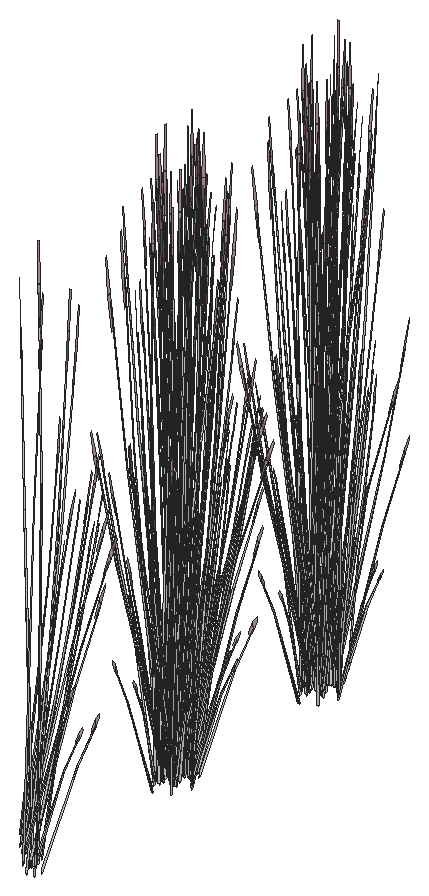
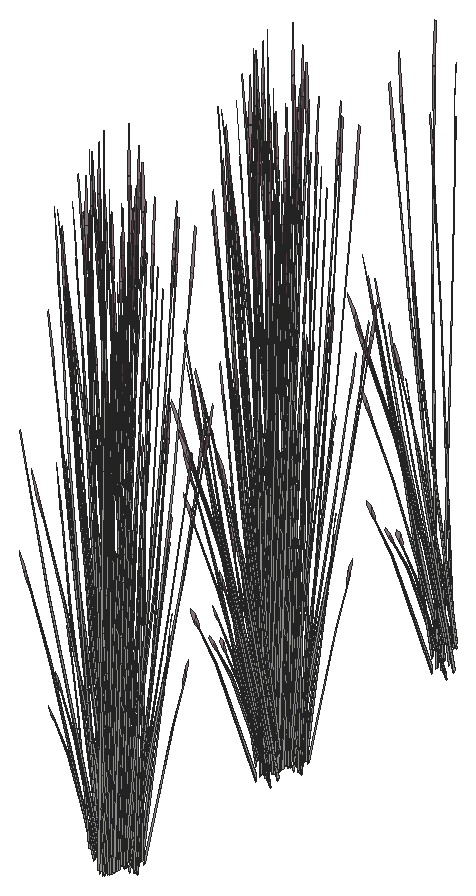
# SketchUp Ruby script. Lengths in inches.
U = 1.inch
M = Sketchup.active_model
def pt(a) = Geom::Point3d.new(a.map { |v| v * U })
def face(e, loops, mat)
  f = e.add_face(loops[0].map { |a| pt(a) })
  loops[1..].each { |l| e.add_face(l.map { |a| pt(a) }).erase! }
  f.material = f.back_material = mat if mat
  f
end
# faces: each face lists its corners as indices into pts; further lists are holes
def faces(e, pts, list, mat = nil) = list.each { |f| face(e, (f[0].is_a?(Array) ? f : [f]).map { |l| l.map { |i| pts[i] } }, mat) }
# xy, xz, yz: faces in a plane at the given z, y or x. An outline is a flat list of corners, or four numbers for a rectangle; further outlines are holes
def ring(l) = l.size == 4 ? [[l[0], l[1]], [l[2], l[1]], [l[2], l[3]], [l[0], l[3]]] : l.each_slice(2).to_a
def flat(e, list, mat, &to3) = list.each { |f| face(e, (f[0].is_a?(Array) ? f : [f]).map { |l| ring(l).map { |u, v| to3.(u, v) } }, mat) }
def xy(e, z, list, mat = nil) = flat(e, list, mat) { |x, y| [x, y, z] }
def xz(e, y, list, mat = nil) = flat(e, list, mat) { |x, z| [x, y, z] }
def yz(e, x, list, mat = nil) = flat(e, list, mat) { |y, z| [x, y, z] }
def lines(e, pts, list) = list.each { |a, b| e.add_line(pt(pts[a]), pt(pts[b])) }
# prism: a flat outline (further loops are holes) pulled along v
def prism(e, loops, v, mat = nil)
  f = face(e, loops, mat); d = Geom::Vector3d.new(v.map { |x| x * U })
  f.pushpull(f.normal.samedirection?(d) ? d.length : -d.length)
end
def box(e, o, s, mat = nil) = prism(e, [[o, [o[0] + s[0], o[1], o[2]], [o[0] + s[0], o[1] + s[1], o[2]], [o[0], o[1] + s[1], o[2]]]], [0, 0, s[2]], mat)
def at(x, y, z, deg = 0) = Geom::Transformation.translation(pt([x, y, z])) * Geom::Transformation.rotation(ORIGIN, Z_AXIS, deg.degrees)
def axes(o, x, y, z) = Geom::Transformation.new([*x, 0, *y, 0, *z, 0, *pt(o).to_a, 1])
def part(name) = M.definitions.add(name)
# library, detail: a bought-in or finely detailed component or shape, given as its bounding box
def library(name, o, s) = part(name).tap { |d| box(d.entities, o, s) }
def detail(e, o, s) = box(e.add_group.entities, o, s)
def put(e, d, t, mat = nil) = e.add_instance(d, t).tap { |i| i.material = mat if mat }
def group(e, t, mat = nil) = e.add_group.tap { |g| g.transformation = t; g.material = mat if mat }.entities
root = M.entities
M.materials.add("LightPink_Translucent").color = [144, 107, 117]
M.materials["LightPink_Translucent"].alpha = 0.75
c1 = part("blade")
p = [[2.15,0.21,22],[0,0.17,0],[0.09,0.45,0],[2.18,0.31,22],[2.29,0.31,22],[0.38,0.45,0],
  [2.48,0.24,33],[2.49,0.24,33],[2.48,0.22,33]]
faces(c1.entities,p,[[0,1,2,3],[4,5,2,3],[6,3,4,7],[8,0,3,6]])
c2 = part("seeds")
p = [[0.3,-0.1,1.38],[-0.01,-0.03,1.59],[-0.01,-0.03,0.03],[0.14,-0.07,-0.07],[0.29,-0.03,3],[0.15,0.01,3.11]]
faces(c2.entities,p,[[0,1,2,3],[1,0,4,5]],"LightPink_Translucent")
c3 = part("blade with seeds")
put(c3.entities,c1,at(0,0,0))
put(c3.entities,c2,axes([2.4,0.25,30.99],[1.5799,-0.05474,1.17369],[-0.12525,1.92788,0.29478],[-0.07173,-0.02425,1.56792]))
put(root,c3,axes([402.59,81.55,2.02],[-0.33032,0.23318,-0.49651],[-0.19744,-0.41812,0],[-0.07523,0.05311,1.57504]))
put(root,c3,axes([403.6875,80.17,2.02],[0,0.46636,-0.49651],[-0.39487,0,0],[0,0.10622,1.57504]))
put(root,c3,axes([402.7,80.22,3.875],[-0.1311,-0.08035,1.71376],[0.27131,-0.33708,0.13857],[0.16909,0.15206,0.73262]))
put(root,c3,axes([403.18,81.13,2.77],[-0.19872,-0.13409,1.1486],[0.2566,-0.13625,0.84392],[0.06921,0.11541,0.25299]))
put(root,c3,axes([402.89,81.48,2.375],[0.22066,0.46731,0],[-0.36918,0.26061,-0.51607],[-0.08408,0.05936,1.63711]))
put(root,c3,axes([403.24,81.63,1.49],[0.02571,-0.06733,1.76342],[0.32373,-0.19829,-0.26939],[0.09815,0.10263,0.30037]))
put(root,c3,axes([402.7,79.625,2.84],[-0.00964,-0.43909,1.41272],[0.43635,0.11382,0.59816],[-0.1032,0.24027,1.3335]))
put(root,c3,axes([402.8125,80.1,2.09],[0.12941,0.42699,-0.69212],[-0.37279,0.15378,-0.18165],[0.0143,0.14459,1.52773]))
put(root,c3,axes([402.74,81.32,4.68],[0.34827,-0.11086,-0.51099],[0.06092,0.41983,-0.3958],[0.09354,0.12031,0.97773]))
put(root,c3,axes([403.22,81.75,2.67],[-0.22633,-0.01463,1.0506],[0.14947,-0.31064,0.58006],[0.08941,0.11036,0.8241]))
put(root,c3,axes([402.48,80.99,2.59],[0.00623,-0.15459,1.43002],[0.29764,-0.17268,-0.30754],[0.09188,0.18503,0.61141]))
put(root,c3,axes([401.73,81.62,1.49],[0.05712,-0.02538,1.76342],[0.34359,0.13968,-0.26939],[0.01005,0.15742,0.30037]))
put(root,c3,axes([401.21,81.21,5],[0.25266,0.31335,-0.5672],[-0.2669,0.27442,-0.43934],[-0.03844,0.15921,1.08528]))
put(root,c3,axes([400.9375,81.68,2.82],[0.32063,-0.08258,0.06507],[0.07371,0.33271,-0.86304],[-0.02033,0.16842,0.7736]))
put(root,c3,axes([401.96,81.51,4.68],[0.34695,0.11691,-0.51099],[-0.11892,0.40083,-0.3958],[0.03181,0.16138,0.97773]))
put(root,c3,axes([402.16,80.6875,3.875],[-0.08068,-0.14973,1.71376],[0.3728,-0.12606,0.13857],[0.08426,0.23506,0.73262]))
put(root,c3,axes([401.8,81.76,4.53],[-0.1064,0.35863,-0.35414],[-0.31043,-0.1046,0.4572],[0.02846,0.14439,0.87481]))
put(root,c3,axes([401.5,80.76,3.875],[-0.00864,-0.17899,1.71376],[0.37441,0.11874,0.13857],[-0.02316,0.25508,0.73262]))
put(root,c3,axes([401.84,81.4375,4.98],[0.16845,0.3792,-0.71045],[-0.34676,0.21133,0.08574],[0.03939,0.18322,1.00501]))
put(root,c3,axes([402.72,99.14,2.59],[-0.10032,0.0944,1.43002],[-0.30046,-0.16522,-0.30754],[0.05569,-0.20547,0.61141]))
put(root,c3,axes([402.27,99.47,4.98],[-0.16845,-0.3792,-0.71045],[0.34676,-0.21133,0.08574],[-0.03939,-0.18322,1.00501]))
put(root,c3,axes([401.98,98.63,1.49],[-0.0592,0.0168,1.76342],[-0.32738,-0.18913,-0.26939],[0.00549,-0.15776,0.30037]))
put(root,c3,axes([402.97,99.84,4.98],[0.00918,-0.43138,-0.71045],[0.38672,0.02897,0.08574],[0.04081,-0.18275,1.00501]))
put(root,c3,axes([402.3,99.15,4.53],[0.1064,-0.35863,-0.35414],[0.31043,0.1046,0.4572],[-0.02846,-0.14439,0.87481]))
put(root,c3,axes([402.53,99.62,3.875],[-0.06572,0.16029,1.71376],[-0.27569,-0.33172,0.13857],[0.12437,-0.20675,0.73262]))
put(root,c3,axes([402.14,99.39,4.68],[-0.34695,-0.11691,-0.51099],[0.11892,-0.40083,-0.3958],[-0.03181,-0.16138,0.97773]))
put(root,c3,axes([402.35,98.39,2.77],[0.04528,0.27194,1.1486],[-0.25117,-0.15062,0.84392],[0.02703,-0.13924,0.25299]))
put(root,c3,axes([402.89,99.7,4.68],[-0.25266,-0.31335,-0.51099],[0.2669,-0.27442,-0.3958],[0.03844,-0.15921,0.97773]))
put(root,c3,axes([403.13,99.58,4.53],[0.23881,-0.24554,-0.35414],[0.22606,0.28036,0.4572],[0.0344,-0.14245,0.87481]))
put(root,c3,axes([401.49,100.89,2.1],[-0.14494,-0.47823,-0.69835],[0.41752,-0.17223,-0.18329],[-0.01602,-0.16194,1.54149]))
put(root,c3,axes([403.43,99.43,1.49],[-0.05283,-0.03674,1.76342],[-0.13569,-0.41045,-0.26939],[0.09154,-0.11138,0.30037]))
put(root,c3,axes([403.42,100.59,4.98],[0.18436,-0.36797,-0.71045],[0.32306,0.26151,0.08574],[0.11008,-0.13332,1.00501]))
put(root,c3,axes([401.43,99.52,2.375],[-0.22066,-0.46731,0],[0.36918,-0.26061,-0.51607],[0.08408,-0.05936,1.63711]))
put(root,c3,axes([403.41,100.42,4.68],[-0.09067,-0.42583,-0.51099],[0.34336,-0.07449,-0.3958],[0.0984,-0.11438,0.97773]))
put(root,c3,axes([401.92,98.96,2.13],[-0.2439,0.26754,-0.03893],[-0.22348,-0.29302,-0.17649],[-0.01573,-0.08303,0.58215]))
put(root,c3,axes([400.63,100.83,2.02],[0,-0.46636,-0.49651],[0.39487,0,0],[0,-0.10622,1.57504]))
put(root,c3,axes([401.73,99.45,2.02],[0.33032,-0.23318,-0.49651],[0.19744,0.41812,0],[0.07523,-0.05311,1.57504]))
put(root,c3,axes([403.69,100.25,2.59],[-0.12609,-0.01381,1.43002],[-0.12917,-0.37055,-0.30754],[0.1549,-0.10482,0.61141]))
put(root,c3,axes([402.12,100.4,2.06],[0.23773,-0.35053,-0.62353],[0.29532,0.31785,-0.16365],[0.09526,-0.08744,1.37633]))
put(root,c3,axes([403.84,99.57,2.77],[-0.11756,0.2374,1.1486],[-0.10105,-0.31895,0.84392],[0.09709,-0.07992,0.25299]))
put(root,c3,axes([403.67,100.46,4.53],[0.30722,-0.06665,-0.35414],[0.08112,0.381,0.4572],[0.08804,-0.10234,0.87481]))
put(root,c3,axes([401.71,101.02,2.21],[0.17124,-0.42022,-0.44739],[0.35581,0.20224,0.21531],[0,-0.09687,1.43643]))
put(root,c3,axes([401.86,100.81,2.67],[-0.04113,-0.53214,-0.29095],[0.42835,-0.03218,-0.50002],[0.07543,-0.07088,1.59708]))
put(root,c3,axes([400.8,100.84,2.03],[0.24637,-0.29097,-0.30978],[0.24637,0.29097,0.30978],[0,-0.09372,1.38974]))
put(root,c3,axes([401.67,101.37,2.67],[-0.39748,-0.22252,-0.29095],[0.19139,-0.46966,-0.50002],[-0.01249,-0.11531,1.59708]))
put(root,c3,axes([401.81,99.63,2.03],[0.32928,0.11539,-0.30978],[-0.08291,0.40636,0.30978],[0.06638,-0.04686,1.38974]))
put(root,c3,axes([401.92,101.23,2.43],[0.39767,0.22603,0.24065],[-0.19139,0.46966,0.50002],[0,-0.10827,1.60543]))
put(root,c3,axes([401.79,100.91,2.72],[-0.38326,0.02879,0.44739],[-0.03466,-0.47788,-0.21531],[0.06861,-0.04843,1.43643]))
put(root,c3,axes([400.8,101.26,2.48],[0,0.46636,0.49651],[-0.39487,0,0],[0,-0.10622,1.57504]))
put(root,c3,axes([403.57,101.36,4.68],[0.09562,-0.42421,-0.51099],[0.32782,0.1454,-0.3958],[0.13199,-0.0389,0.97773]))
put(root,c3,axes([403.06,99.64,2.375],[0.22066,-0.46731,0],[0.36918,0.26061,-0.51607],[0.08408,0.05936,1.63711]))
put(root,c3,axes([401.78,101.08,2.36],[0.15345,0.52148,0.45755],[-0.43845,0.18134,0.17955],[0.00536,-0.09582,1.58856]))
put(root,c3,axes([403.92,101.48,1.98],[-0.22732,0.05597,1.41583],[-0.03618,-0.44548,0.08104],[0.15921,-0.06743,0.80566]))
put(root,c3,axes([404.34,101.09,2.26],[-0.21881,-0.29821,-0.06488],[0.23965,-0.27324,-0.29416],[0.0679,-0.01924,0.97024]))
put(root,c3,axes([401.7,101.5,2.72],[-0.17124,0.42022,0.44739],[-0.35581,-0.20224,-0.21531],[0,-0.09687,1.43643]))
put(root,c3,axes([402.33,101.13,2.21],[0,-0.53961,0],[0.44133,0,0],[0,0,1.79456]))
put(root,c3,axes([402.87,99.88,2.48],[-0.33032,-0.23318,0.49651],[0.19744,-0.41812,0],[0.07523,0.05311,1.57504]))
put(root,c3,axes([403.51,101.52,4.98],[0.31014,-0.20596,-0.71045],[0.17284,0.42397,0.08574],[0.14985,-0.04816,1.00501]))
put(root,c3,axes([402.12,100.79,2.36],[-0.29264,0.42323,0.45755],[-0.34767,-0.3736,0.17955],[0.07055,-0.04224,1.58856]))
put(root,c3,axes([402.44,101.55,2.3],[-0.32829,-0.4014,-0.06131],[0.32849,-0.40164,0],[-0.01146,-0.01402,1.75571]))
put(root,c3,axes([401.61,100.09,2.47],[-0.10196,0.46348,0.17642],[-0.3731,-0.13116,0.35086],[0.06445,-0.00226,1.60407]))
put(root,c3,axes([401.46,100.47,1.59],[-0.3474,0.18671,1.28929],[-0.11057,-0.53572,0.50096],[0.21332,0.00891,1.46642]))
put(root,c3,axes([402.39,100.61,2.62],[0.06809,-0.4162,0.1448],[0.33266,0.07225,-0.41347],[0.06054,0.04274,1.26744]))
put(root,c3,axes([401.82,101.6,2.36],[0.44609,0.09826,0.45755],[-0.09078,0.55493,0.17955],[-0.06519,-0.05359,1.58856]))
put(root,c3,axes([404.17,101.19,1.49],[-0.01845,-0.0708,1.76342],[0.12793,-0.41416,-0.26939],[0.12905,-0.00596,0.30037]))
put(root,c3,axes([402.25,100.72,2.72],[-0.21202,-0.39143,0.44739],[0.32115,-0.27564,-0.21531],[0.06861,0.04843,1.43643]))
put(root,c3,axes([401.58,102.48,2.47],[0.37926,-0.12378,0.17642],[0.09365,0.46065,0.35086],[-0.03382,-0.06712,1.60407]))
put(root,c3,axes([402.36,100.74,2.67],[0.35635,-0.30962,-0.29095],[0.23697,0.43749,-0.50002],[0.08792,0.04443,1.59708]))
put(root,c3,axes([403.78,101.56,4.53],[0.29332,0.1301,-0.35414],[-0.08555,0.37955,0.4572],[0.11809,-0.0348,0.87481]))
put(root,c3,axes([403.26,99.92,2.02],[0.33032,0.23318,-0.49651],[-0.19744,0.41812,0],[0.07523,0.05311,1.57504]))
put(root,c3,axes([402.63,101.25,2.21],[0.39487,0,0],[0,0.48281,0],[0,0,1.78407]))
put(root,c3,axes([402.74,100.12,2.47],[-0.37926,0.12378,0.17642],[-0.09365,-0.46065,0.35086],[0.03382,0.06712,1.60407]))
put(root,c3,axes([402.98,101.09,3.875],[-0.14639,0.01056,1.71376],[0.09712,-0.45778,0.13857],[0.20862,0.02831,0.73262]))
put(root,c3,axes([403.17,100.09,2.03],[0.08291,0.40636,-0.30978],[-0.32928,0.11539,0.30978],[0.06638,0.04686,1.38974]))
put(root,c3,axes([402.5,101,2.38],[-0.44609,-0.09826,0.49198],[0.09078,-0.55493,0.19306],[0.06519,0.05359,1.70813]))
put(root,c3,axes([402.15,102.375,2.2],[-0.11516,-0.40207,0],[0.32884,-0.1408,0],[0,0,1.54371]))
put(root,c3,axes([401.93,101.99,2.62],[-0.06809,0.4162,0.1448],[-0.33266,-0.07225,-0.41347],[-0.06054,-0.04274,1.26744]))
put(root,c3,axes([402.58,102.32,2.18],[0.37054,-0.15823,-0.19198],[0.1302,0.45581,0.00008],[0.0409,-0.01749,1.73897]))
put(root,c3,axes([402.71,102.51,2.47],[0.10196,-0.46348,0.17642],[0.3731,0.13116,0.35086],[-0.06445,0.00226,1.60407]))
put(root,c3,axes([402.62,101.46,2.21],[0.24637,0.30123,0],[-0.24637,0.30123,0],[0,0,1.69266]))
put(root,c3,axes([403.29,101.32,2.47],[-0.2773,-0.3397,0.17642],[0.27945,-0.32949,0.35086],[-0.03063,0.06937,1.60407]))
put(root,c3,axes([402.78,100.8125,2.06],[0.36714,0.07646,-0.62353],[-0.07747,0.47163,-0.16365],[0.10956,0.05715,1.37633]))
put(root,c3,axes([404.4,101.64,2.77],[-0.21807,0.07699,1.1486],[0.10265,-0.31819,0.84392],[0.11568,0.02177,0.25299]))
put(root,c3,axes([402.07,102.56,2.2],[-0.35581,-0.20937,0],[0.17124,-0.43505,0],[0,0,1.62707]))
put(root,c3,axes([402.62,101.1,2.72],[0.17124,-0.42022,0.44739],[0.35581,0.20224,-0.21531],[0,0.09687,1.43643]))
put(root,c3,axes([402.55,101.34,2.29],[0,0.53934,-0.05637],[-0.44133,0,0],[0,0.01695,1.79368]))
put(root,c3,axes([402.58,100.96,2.21],[0.21202,0.39143,-0.44739],[-0.32115,0.27564,0.21531],[0.06861,0.04843,1.43643]))
put(root,c3,axes([404.02,102.62,3.93],[-0.06755,-0.39203,-0.03492],[0.31928,-0.09013,-0.15832],[0.06667,0.02485,0.52218]))
put(root,c3,axes([403.52,101.34,2.48],[0,-0.46636,0.49651],[0.39487,0,0],[0,0.10622,1.57504]))
put(root,c3,axes([402.53,101.6875,2.72],[0.38326,-0.02879,0.44739],[0.03466,0.47788,-0.21531],[-0.06861,0.04843,1.43643]))
put(root,c3,axes([402.77,101.2,2.62],[0.32884,-0.136,0.1448],[0.11516,0.38837,-0.41347],[0,0.08547,1.26744]))
put(root,c3,axes([403.99,102.15,2.59],[-0.085,-0.1147,1.43002],[0.1106,-0.37943,-0.30754],[0.17198,0.0514,0.61141]))
put(root,c3,axes([402.47,102.5625,2.2],[0.35581,0.20937,0],[-0.17124,0.43505,0],[0,0,1.74954]))
put(root,c3,axes([402.61,103.03,2.19],[-0.21791,-0.46895,-0.05142],[0.36918,-0.26061,0.51607],[-0.09097,0.04465,1.6363]))
put(root,c3,axes([402.53,101.89,2.62],[0.26075,0.2802,0.1448],[-0.2175,0.31612,-0.41347],[-0.06054,0.04274,1.26744]))
put(root,c3,axes([403.21,102.38,4.98],[0.35281,0.01123,-0.71045],[-0.0237,0.47284,0.08574],[0.14947,0.0499,1.00501]))
put(root,c3,axes([402.8125,102.76,2.48],[0.33032,-0.23318,0.49651],[0.19744,0.41812,0],[-0.07523,0.05311,1.57504]))
put(root,c3,axes([402.34,102.39,2.29],[0.15345,0.53576,-0.06012],[-0.43845,0.18773,0],[0.00536,0.01871,1.72173]))
put(root,c3,axes([402.51,102.97,2.03],[-0.32928,-0.11539,-0.30978],[0.08291,-0.40636,0.30978],[-0.06638,0.04686,1.38974]))
put(root,c3,axes([403.78,101.42,2.375],[0.44133,0,0],[0,0.52122,-0.51607],[0,0.11871,1.63711]))
put(root,c3,axes([403.61,101.69,2.2],[-0.44111,-0.00373,-0.04976],[0,-0.52122,0.49943],[-0.01386,0.11865,1.58352]))
put(root,c3,axes([402.65,101.23,2.67],[0.39748,0.22252,-0.29095],[-0.19139,0.46966,-0.50002],[0.01249,0.11531,1.59708]))
put(root,c3,axes([403.42,102.57,4.53],[0.20082,0.29199,-0.35414],[-0.2293,0.2764,0.4572],[0.1165,0.04206,0.87481]))
put(root,c3,axes([403.52,101.76,2.03],[-0.24637,0.29097,-0.30978],[-0.24637,-0.29097,0.30978],[0,0.09372,1.38974]))
put(root,c3,axes([402.46,101.79,2.67],[0.04113,0.53214,-0.29095],[-0.42835,0.03218,-0.50002],[-0.07543,0.07088,1.59708]))
put(root,c3,axes([402.61,101.58,2.21],[-0.17124,0.42022,-0.44739],[-0.35581,-0.20224,0.21531],[0,0.09687,1.43643]))
put(root,c3,axes([402.62,102.79,2.33],[0.44186,0.15158,0.30756],[-0.11054,0.54181,-0.36492],[-0.07313,0.06781,1.64885]))
put(root,c3,axes([402.59,103.15,2.02],[-0.33032,0.23318,-0.49651],[-0.19744,-0.41812,0],[-0.07523,0.05311,1.57504]))
put(root,c3,axes([403.6875,101.77,2.02],[0,0.46636,-0.49651],[-0.39487,0,0],[0,0.10622,1.57504]))
put(root,c3,axes([402.7,101.82,3.875],[-0.1311,-0.08035,1.71376],[0.27131,-0.33708,0.13857],[0.16909,0.15206,0.73262]))
put(root,c3,axes([403.18,102.74,2.77],[-0.19872,-0.13409,1.1486],[0.2566,-0.13625,0.84392],[0.06921,0.11541,0.25299]))
put(root,c3,axes([402.89,103.08,2.375],[0.22066,0.46731,0],[-0.36918,0.26061,-0.51607],[-0.08408,0.05936,1.63711]))
put(root,c3,axes([403.24,103.24,1.49],[0.02571,-0.06733,1.76342],[0.32373,-0.19829,-0.26939],[0.09815,0.10263,0.30037]))
put(root,c3,axes([402.7,101.23,2.84],[-0.00964,-0.43909,1.41272],[0.43635,0.11382,0.59816],[-0.1032,0.24027,1.3335]))
put(root,c3,axes([402.8125,101.71,2.09],[0.12941,0.42699,-0.69212],[-0.37279,0.15378,-0.18165],[0.0143,0.14459,1.52773]))
put(root,c3,axes([402.74,102.92,4.68],[0.34827,-0.11086,-0.51099],[0.06092,0.41983,-0.3958],[0.09354,0.12031,0.97773]))
put(root,c3,axes([403.22,103.35,2.67],[-0.22633,-0.01463,1.0506],[0.14947,-0.31064,0.58006],[0.08941,0.11036,0.8241]))
put(root,c3,axes([402.48,102.6,2.59],[0.00623,-0.15459,1.43002],[0.29764,-0.17268,-0.30754],[0.09188,0.18503,0.61141]))
put(root,c3,axes([401.73,103.22,1.49],[0.05712,-0.02538,1.76342],[0.34359,0.13968,-0.26939],[0.01005,0.15742,0.30037]))
put(root,c3,axes([401.21,102.8125,5],[0.25266,0.31335,-0.5672],[-0.2669,0.27442,-0.43934],[-0.03844,0.15921,1.08528]))
put(root,c3,axes([400.9375,103.28,2.82],[0.32063,-0.08258,0.06507],[0.07371,0.33271,-0.86304],[-0.02033,0.16842,0.7736]))
put(root,c3,axes([401.96,103.12,4.68],[0.34695,0.11691,-0.51099],[-0.11892,0.40083,-0.3958],[0.03181,0.16138,0.97773]))
put(root,c3,axes([402.16,102.29,3.875],[-0.08068,-0.14973,1.71376],[0.3728,-0.12606,0.13857],[0.08426,0.23506,0.73262]))
put(root,c3,axes([401.8,103.36,4.53],[-0.1064,0.35863,-0.35414],[-0.31043,-0.1046,0.4572],[0.02846,0.14439,0.87481]))
put(root,c3,axes([401.5,102.37,3.875],[-0.00864,-0.17899,1.71376],[0.37441,0.11874,0.13857],[-0.02316,0.25508,0.73262]))
put(root,c3,axes([401.84,103.04,4.98],[0.16845,0.3792,-0.71045],[-0.34676,0.21133,0.08574],[0.03939,0.18322,1.00501]))
put(root,c3,axes([402.72,119.23,2.59],[-0.10032,0.0944,1.43002],[-0.30046,-0.16522,-0.30754],[0.05569,-0.20547,0.61141]))
put(root,c3,axes([402.27,119.5625,4.98],[-0.16845,-0.3792,-0.71045],[0.34676,-0.21133,0.08574],[-0.03939,-0.18322,1.00501]))
put(root,c3,axes([401.98,118.72,1.49],[-0.0592,0.0168,1.76342],[-0.32738,-0.18913,-0.26939],[0.00549,-0.15776,0.30037]))
put(root,c3,axes([402.97,119.93,4.98],[0.00918,-0.43138,-0.71045],[0.38672,0.02897,0.08574],[0.04081,-0.18275,1.00501]))
put(root,c3,axes([402.3,119.24,4.53],[0.1064,-0.35863,-0.35414],[0.31043,0.1046,0.4572],[-0.02846,-0.14439,0.87481]))
put(root,c3,axes([402.53,119.71,3.875],[-0.06572,0.16029,1.71376],[-0.27569,-0.33172,0.13857],[0.12437,-0.20675,0.73262]))
put(root,c3,axes([402.14,119.49,4.68],[-0.34695,-0.11691,-0.51099],[0.11892,-0.40083,-0.3958],[-0.03181,-0.16138,0.97773]))
put(root,c3,axes([402.35,118.48,2.77],[0.04528,0.27194,1.1486],[-0.25117,-0.15062,0.84392],[0.02703,-0.13924,0.25299]))
put(root,c3,axes([402.89,119.79,4.68],[-0.25266,-0.31335,-0.51099],[0.2669,-0.27442,-0.3958],[0.03844,-0.15921,0.97773]))
put(root,c3,axes([403.13,119.67,4.53],[0.23881,-0.24554,-0.35414],[0.22606,0.28036,0.4572],[0.0344,-0.14245,0.87481]))
put(root,c3,axes([401.49,120.99,2.1],[-0.14494,-0.47823,-0.69835],[0.41752,-0.17223,-0.18329],[-0.01602,-0.16194,1.54149]))
put(root,c3,axes([403.43,119.53,1.49],[-0.05283,-0.03674,1.76342],[-0.13569,-0.41045,-0.26939],[0.09154,-0.11138,0.30037]))
put(root,c3,axes([403.42,120.68,4.98],[0.18436,-0.36797,-0.71045],[0.32306,0.26151,0.08574],[0.11008,-0.13332,1.00501]))
put(root,c3,axes([401.43,119.61,2.375],[-0.22066,-0.46731,0],[0.36918,-0.26061,-0.51607],[0.08408,-0.05936,1.63711]))
put(root,c3,axes([403.41,120.51,4.68],[-0.09067,-0.42583,-0.51099],[0.34336,-0.07449,-0.3958],[0.0984,-0.11438,0.97773]))
put(root,c3,axes([401.92,119.05,2.13],[-0.2439,0.26754,-0.03893],[-0.22348,-0.29302,-0.17649],[-0.01573,-0.08303,0.58215]))
put(root,c3,axes([400.63,120.92,2.02],[0,-0.46636,-0.49651],[0.39487,0,0],[0,-0.10622,1.57504]))
put(root,c3,axes([401.73,119.54,2.02],[0.33032,-0.23318,-0.49651],[0.19744,0.41812,0],[0.07523,-0.05311,1.57504]))
put(root,c3,axes([403.69,120.35,2.59],[-0.12609,-0.01381,1.43002],[-0.12917,-0.37055,-0.30754],[0.1549,-0.10482,0.61141]))
put(root,c3,axes([402.12,120.5,2.06],[0.23773,-0.35053,-0.62353],[0.29532,0.31785,-0.16365],[0.09526,-0.08744,1.37633]))
put(root,c3,axes([403.84,119.66,2.77],[-0.11756,0.2374,1.1486],[-0.10105,-0.31895,0.84392],[0.09709,-0.07992,0.25299]))
put(root,c3,axes([403.67,120.56,4.53],[0.30722,-0.06665,-0.35414],[0.08112,0.381,0.4572],[0.08804,-0.10234,0.87481]))
put(root,c3,axes([401.71,121.11,2.21],[0.17124,-0.42022,-0.44739],[0.35581,0.20224,0.21531],[0,-0.09687,1.43643]))
put(root,c3,axes([401.86,120.9,2.67],[-0.04113,-0.53214,-0.29095],[0.42835,-0.03218,-0.50002],[0.07543,-0.07088,1.59708]))
put(root,c3,axes([400.8,120.93,2.03],[0.24637,-0.29097,-0.30978],[0.24637,0.29097,0.30978],[0,-0.09372,1.38974]))
put(root,c3,axes([401.67,121.46,2.67],[-0.39748,-0.22252,-0.29095],[0.19139,-0.46966,-0.50002],[-0.01249,-0.11531,1.59708]))
put(root,c3,axes([401.81,119.72,2.03],[0.32928,0.11539,-0.30978],[-0.08291,0.40636,0.30978],[0.06638,-0.04686,1.38974]))
put(root,c3,axes([401.92,121.32,2.43],[0.39767,0.22603,0.24065],[-0.19139,0.46966,0.50002],[0,-0.10827,1.60543]))
put(root,c3,axes([401.79,121,2.72],[-0.38326,0.02879,0.44739],[-0.03466,-0.47788,-0.21531],[0.06861,-0.04843,1.43643]))
put(root,c3,axes([400.8,121.35,2.48],[0,0.46636,0.49651],[-0.39487,0,0],[0,-0.10622,1.57504]))
put(root,c3,axes([403.57,121.46,4.68],[0.09562,-0.42421,-0.51099],[0.32782,0.1454,-0.3958],[0.13199,-0.0389,0.97773]))
put(root,c3,axes([403.06,119.73,2.375],[0.22066,-0.46731,0],[0.36918,0.26061,-0.51607],[0.08408,0.05936,1.63711]))
put(root,c3,axes([401.78,121.18,2.36],[0.15345,0.52148,0.45755],[-0.43845,0.18134,0.17955],[0.00536,-0.09582,1.58856]))
put(root,c3,axes([403.92,121.58,1.98],[-0.22732,0.05597,1.41583],[-0.03618,-0.44548,0.08104],[0.15921,-0.06743,0.80566]))
put(root,c3,axes([404.34,121.18,2.26],[-0.21881,-0.29821,-0.06488],[0.23965,-0.27324,-0.29416],[0.0679,-0.01924,0.97024]))
put(root,c3,axes([401.7,121.59,2.72],[-0.17124,0.42022,0.44739],[-0.35581,-0.20224,-0.21531],[0,-0.09687,1.43643]))
put(root,c3,axes([402.33,121.22,2.21],[0,-0.53961,0],[0.44133,0,0],[0,0,1.79456]))
put(root,c3,axes([402.87,119.97,2.48],[-0.33032,-0.23318,0.49651],[0.19744,-0.41812,0],[0.07523,0.05311,1.57504]))
put(root,c3,axes([403.51,121.61,4.98],[0.31014,-0.20596,-0.71045],[0.17284,0.42397,0.08574],[0.14985,-0.04816,1.00501]))
put(root,c3,axes([402.12,120.88,2.36],[-0.29264,0.42323,0.45755],[-0.34767,-0.3736,0.17955],[0.07055,-0.04224,1.58856]))
put(root,c3,axes([402.44,121.64,2.3],[-0.32829,-0.4014,-0.06131],[0.32849,-0.40164,0],[-0.01146,-0.01402,1.75571]))
put(root,c3,axes([401.61,120.18,2.47],[-0.10196,0.46348,0.17642],[-0.3731,-0.13116,0.35086],[0.06445,-0.00226,1.60407]))
put(root,c3,axes([401.46,120.56,1.59],[-0.3474,0.18671,1.28929],[-0.11057,-0.53572,0.50096],[0.21332,0.00891,1.46642]))
put(root,c3,axes([402.39,120.7,2.62],[0.06809,-0.4162,0.1448],[0.33266,0.07225,-0.41347],[0.06054,0.04274,1.26744]))
put(root,c3,axes([401.82,121.6875,2.36],[0.44609,0.09826,0.45755],[-0.09078,0.55493,0.17955],[-0.06519,-0.05359,1.58856]))
put(root,c3,axes([404.17,121.29,1.49],[-0.01845,-0.0708,1.76342],[0.12793,-0.41416,-0.26939],[0.12905,-0.00596,0.30037]))
put(root,c3,axes([402.25,120.81,2.72],[-0.21202,-0.39143,0.44739],[0.32115,-0.27564,-0.21531],[0.06861,0.04843,1.43643]))
put(root,c3,axes([401.58,122.57,2.47],[0.37926,-0.12378,0.17642],[0.09365,0.46065,0.35086],[-0.03382,-0.06712,1.60407]))
put(root,c3,axes([402.36,120.83,2.67],[0.35635,-0.30962,-0.29095],[0.23697,0.43749,-0.50002],[0.08792,0.04443,1.59708]))
put(root,c3,axes([403.78,121.65,4.53],[0.29332,0.1301,-0.35414],[-0.08555,0.37955,0.4572],[0.11809,-0.0348,0.87481]))
put(root,c3,axes([403.26,120.01,2.02],[0.33032,0.23318,-0.49651],[-0.19744,0.41812,0],[0.07523,0.05311,1.57504]))
put(root,c3,axes([402.63,121.34,2.21],[0.39487,0,0],[0,0.48281,0],[0,0,1.78407]))
put(root,c3,axes([402.74,120.21,2.47],[-0.37926,0.12378,0.17642],[-0.09365,-0.46065,0.35086],[0.03382,0.06712,1.60407]))
put(root,c3,axes([402.98,121.18,3.875],[-0.14639,0.01056,1.71376],[0.09712,-0.45778,0.13857],[0.20862,0.02831,0.73262]))
put(root,c3,axes([403.17,120.19,2.03],[0.08291,0.40636,-0.30978],[-0.32928,0.11539,0.30978],[0.06638,0.04686,1.38974]))
put(root,c3,axes([402.5,121.1,2.38],[-0.44609,-0.09826,0.49198],[0.09078,-0.55493,0.19306],[0.06519,0.05359,1.70813]))
put(root,c3,axes([402.15,122.47,2.2],[-0.11516,-0.40207,0],[0.32884,-0.1408,0],[0,0,1.54371]))
put(root,c3,axes([401.93,122.08,2.62],[-0.06809,0.4162,0.1448],[-0.33266,-0.07225,-0.41347],[-0.06054,-0.04274,1.26744]))
put(root,c3,axes([402.58,122.41,2.18],[0.37054,-0.15823,-0.19198],[0.1302,0.45581,0.00008],[0.0409,-0.01749,1.73897]))
put(root,c3,axes([402.71,122.6,2.47],[0.10196,-0.46348,0.17642],[0.3731,0.13116,0.35086],[-0.06445,0.00226,1.60407]))
put(root,c3,axes([402.62,121.55,2.21],[0.24637,0.30123,0],[-0.24637,0.30123,0],[0,0,1.69266]))
put(root,c3,axes([403.29,121.42,2.47],[-0.2773,-0.3397,0.17642],[0.27945,-0.32949,0.35086],[-0.03063,0.06937,1.60407]))
put(root,c3,axes([402.78,120.9,2.06],[0.36714,0.07646,-0.62353],[-0.07747,0.47163,-0.16365],[0.10956,0.05715,1.37633]))
put(root,c3,axes([404.4,121.73,2.77],[-0.21807,0.07699,1.1486],[0.10265,-0.31819,0.84392],[0.11568,0.02177,0.25299]))
put(root,c3,axes([402.07,122.65,2.2],[-0.35581,-0.20937,0],[0.17124,-0.43505,0],[0,0,1.62707]))
put(root,c3,axes([402.62,121.2,2.72],[0.17124,-0.42022,0.44739],[0.35581,0.20224,-0.21531],[0,0.09687,1.43643]))
put(root,c3,axes([402.55,121.4375,2.29],[0,0.53934,-0.05637],[-0.44133,0,0],[0,0.01695,1.79368]))
put(root,c3,axes([402.58,121.05,2.21],[0.21202,0.39143,-0.44739],[-0.32115,0.27564,0.21531],[0.06861,0.04843,1.43643]))
put(root,c3,axes([404.02,122.71,3.93],[-0.06755,-0.39203,-0.03492],[0.31928,-0.09013,-0.15832],[0.06667,0.02485,0.52218]))
put(root,c3,axes([403.52,121.43,2.48],[0,-0.46636,0.49651],[0.39487,0,0],[0,0.10622,1.57504]))
put(root,c3,axes([402.53,121.78,2.72],[0.38326,-0.02879,0.44739],[0.03466,0.47788,-0.21531],[-0.06861,0.04843,1.43643]))
put(root,c3,axes([402.77,121.29,2.62],[0.32884,-0.136,0.1448],[0.11516,0.38837,-0.41347],[0,0.08547,1.26744]))
put(root,c3,axes([403.99,122.24,2.59],[-0.085,-0.1147,1.43002],[0.1106,-0.37943,-0.30754],[0.17198,0.0514,0.61141]))
put(root,c3,axes([402.47,122.66,2.2],[0.35581,0.20937,0],[-0.17124,0.43505,0],[0,0,1.74954]))
put(root,c3,axes([402.61,123.12,2.19],[-0.21791,-0.46895,-0.05142],[0.36918,-0.26061,0.51607],[-0.09097,0.04465,1.6363]))
put(root,c3,axes([402.53,121.98,2.62],[0.26075,0.2802,0.1448],[-0.2175,0.31612,-0.41347],[-0.06054,0.04274,1.26744]))
put(root,c3,axes([403.21,122.47,4.98],[0.35281,0.01123,-0.71045],[-0.0237,0.47284,0.08574],[0.14947,0.0499,1.00501]))
put(root,c3,axes([402.8125,122.85,2.48],[0.33032,-0.23318,0.49651],[0.19744,0.41812,0],[-0.07523,0.05311,1.57504]))
put(root,c3,axes([402.34,122.48,2.29],[0.15345,0.53576,-0.06012],[-0.43845,0.18773,0],[0.00536,0.01871,1.72173]))
put(root,c3,axes([402.51,123.06,2.03],[-0.32928,-0.11539,-0.30978],[0.08291,-0.40636,0.30978],[-0.06638,0.04686,1.38974]))
put(root,c3,axes([403.78,121.51,2.375],[0.44133,0,0],[0,0.52122,-0.51607],[0,0.11871,1.63711]))
put(root,c3,axes([403.61,121.78,2.2],[-0.44111,-0.00373,-0.04976],[0,-0.52122,0.49943],[-0.01386,0.11865,1.58352]))
put(root,c3,axes([402.65,121.32,2.67],[0.39748,0.22252,-0.29095],[-0.19139,0.46966,-0.50002],[0.01249,0.11531,1.59708]))
